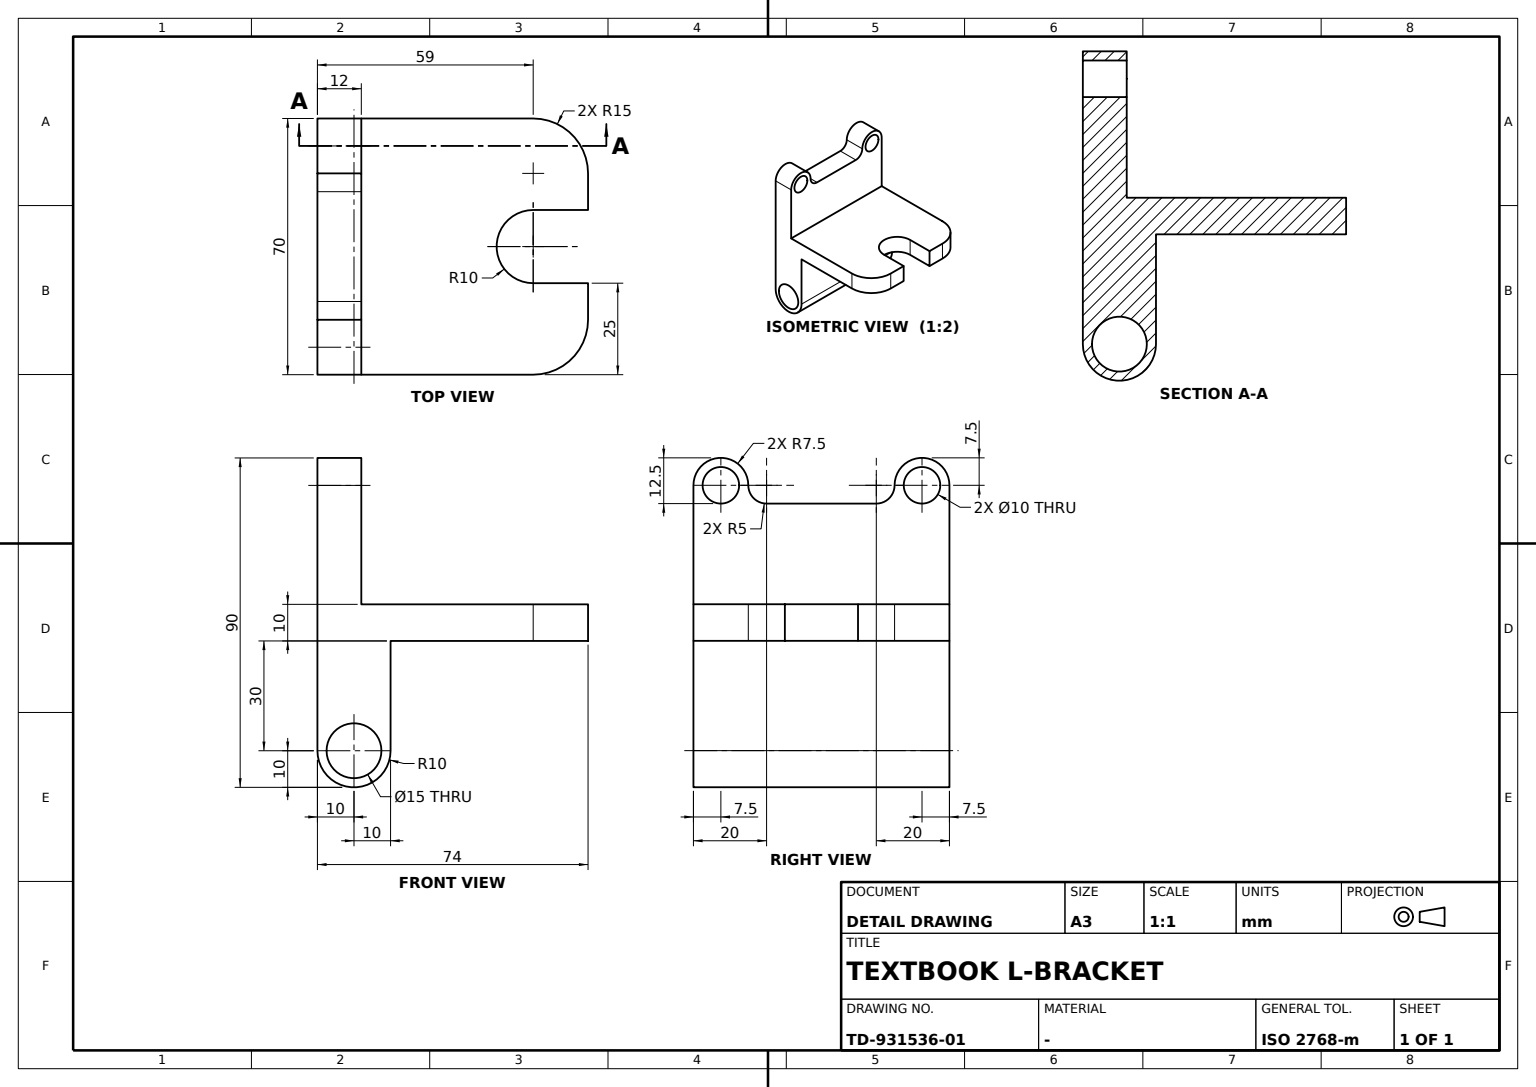
ISO-10303-21;
HEADER;
FILE_DESCRIPTION((''),'2;1');
FILE_NAME('','',(''),(''),'','','');
FILE_SCHEMA(('AUTOMOTIVE_DESIGN'));
ENDSEC;
DATA;
#1=APPLICATION_CONTEXT('');
#2=PRODUCT_CONTEXT('',#1,'mechanical');
#3=PRODUCT('','','',(#2));
#4=PRODUCT_DEFINITION_FORMATION('','',#3);
#5=PRODUCT_DEFINITION_CONTEXT('',#1,'design');
#6=PRODUCT_DEFINITION('','',#4,#5);
#7=PRODUCT_DEFINITION_SHAPE('','',#6);
#8=(LENGTH_UNIT()NAMED_UNIT(*)SI_UNIT(.MILLI.,.METRE.));
#9=(NAMED_UNIT(*)PLANE_ANGLE_UNIT()SI_UNIT($,.RADIAN.));
#10=(NAMED_UNIT(*)SI_UNIT($,.STERADIAN.)SOLID_ANGLE_UNIT());
#11=UNCERTAINTY_MEASURE_WITH_UNIT(LENGTH_MEASURE(1.E-05),#8,'distance_accuracy_value','');
#12=(GEOMETRIC_REPRESENTATION_CONTEXT(3)GLOBAL_UNCERTAINTY_ASSIGNED_CONTEXT((#11))GLOBAL_UNIT_ASSIGNED_CONTEXT((#8,#9,#10))REPRESENTATION_CONTEXT('',''));
#13=CARTESIAN_POINT('',(20.,-6.,37.5));
#14=VERTEX_POINT('',#13);
#15=CARTESIAN_POINT('',(20.,6.,37.5));
#16=VERTEX_POINT('',#15);
#17=CARTESIAN_POINT('',(20.,0.,37.5));
#18=DIRECTION('',(0.,1.,0.));
#19=VECTOR('',#18,1000.);
#20=LINE('',#17,#19);
#21=EDGE_CURVE('',#14,#16,#20,.T.);
#22=ORIENTED_EDGE('',*,*,#21,.F.);
#23=CARTESIAN_POINT('',(35.,-6.,37.5));
#24=VERTEX_POINT('',#23);
#25=CARTESIAN_POINT('',(27.5,-6.,37.5));
#26=DIRECTION('',(-1.,0.,0.));
#27=AXIS2_PLACEMENT_3D('',#25,#18,#26);
#28=CIRCLE('',#27,7.5);
#29=EDGE_CURVE('',#14,#24,#28,.T.);
#30=ORIENTED_EDGE('',*,*,#29,.T.);
#31=CARTESIAN_POINT('',(35.,6.,37.5));
#32=VERTEX_POINT('',#31);
#33=CARTESIAN_POINT('',(35.,0.,37.5));
#34=DIRECTION('',(0.,-1.,0.));
#35=VECTOR('',#34,1000.);
#36=LINE('',#33,#35);
#37=EDGE_CURVE('',#32,#24,#36,.T.);
#38=ORIENTED_EDGE('',*,*,#37,.F.);
#39=CARTESIAN_POINT('',(27.5,6.,37.5));
#40=AXIS2_PLACEMENT_3D('',#39,#18,#26);
#41=CIRCLE('',#40,7.5);
#42=EDGE_CURVE('',#16,#32,#41,.T.);
#43=ORIENTED_EDGE('',*,*,#42,.F.);
#44=EDGE_LOOP('',(#22,#30,#38,#43));
#45=FACE_OUTER_BOUND('',#44,.T.);
#46=CARTESIAN_POINT('',(27.5,0.,37.5));
#47=AXIS2_PLACEMENT_3D('',#46,#34,#26);
#48=CYLINDRICAL_SURFACE('',#47,7.5);
#49=ADVANCED_FACE('',(#45),#48,.T.);
#50=CARTESIAN_POINT('',(-32.5,-6.,37.5));
#51=VERTEX_POINT('',#50);
#52=CARTESIAN_POINT('',(-22.5,-6.,37.5));
#53=VERTEX_POINT('',#52);
#54=CARTESIAN_POINT('',(-27.5,-6.,37.5));
#55=AXIS2_PLACEMENT_3D('',#54,#18,#26);
#56=CIRCLE('',#55,5.);
#57=EDGE_CURVE('',#51,#53,#56,.T.);
#58=ORIENTED_EDGE('',*,*,#57,.F.);
#59=CARTESIAN_POINT('',(-32.5,6.,37.5));
#60=VERTEX_POINT('',#59);
#61=CARTESIAN_POINT('',(-32.5,0.,37.5));
#62=LINE('',#61,#35);
#63=EDGE_CURVE('',#60,#51,#62,.T.);
#64=ORIENTED_EDGE('',*,*,#63,.F.);
#65=CARTESIAN_POINT('',(-22.5,6.,37.5));
#66=VERTEX_POINT('',#65);
#67=CARTESIAN_POINT('',(-27.5,6.,37.5));
#68=AXIS2_PLACEMENT_3D('',#67,#18,#26);
#69=CIRCLE('',#68,5.);
#70=EDGE_CURVE('',#60,#66,#69,.T.);
#71=ORIENTED_EDGE('',*,*,#70,.T.);
#72=CARTESIAN_POINT('',(-22.5,0.,37.5));
#73=LINE('',#72,#35);
#74=EDGE_CURVE('',#66,#53,#73,.T.);
#75=ORIENTED_EDGE('',*,*,#74,.T.);
#76=EDGE_LOOP('',(#58,#64,#71,#75));
#77=FACE_OUTER_BOUND('',#76,.T.);
#78=CARTESIAN_POINT('',(-27.5,0.,37.5));
#79=AXIS2_PLACEMENT_3D('',#78,#34,#26);
#80=CYLINDRICAL_SURFACE('',#79,5.);
#81=ADVANCED_FACE('',(#77),#80,.F.);
#82=CARTESIAN_POINT('',(15.,-6.,32.5));
#83=VERTEX_POINT('',#82);
#84=CARTESIAN_POINT('',(15.,6.,32.5));
#85=VERTEX_POINT('',#84);
#86=CARTESIAN_POINT('',(15.,0.,32.5));
#87=LINE('',#86,#19);
#88=EDGE_CURVE('',#83,#85,#87,.T.);
#89=ORIENTED_EDGE('',*,*,#88,.T.);
#90=CARTESIAN_POINT('',(-15.,6.,32.5));
#91=VERTEX_POINT('',#90);
#92=CARTESIAN_POINT('',(0.,6.,32.5));
#93=VECTOR('',#26,1000.);
#94=LINE('',#92,#93);
#95=EDGE_CURVE('',#85,#91,#94,.T.);
#96=ORIENTED_EDGE('',*,*,#95,.T.);
#97=CARTESIAN_POINT('',(-15.,-6.,32.5));
#98=VERTEX_POINT('',#97);
#99=CARTESIAN_POINT('',(-15.,0.,32.5));
#100=LINE('',#99,#19);
#101=EDGE_CURVE('',#98,#91,#100,.T.);
#102=ORIENTED_EDGE('',*,*,#101,.F.);
#103=CARTESIAN_POINT('',(0.,-6.,32.5));
#104=DIRECTION('',(1.,0.,0.));
#105=VECTOR('',#104,1000.);
#106=LINE('',#103,#105);
#107=EDGE_CURVE('',#98,#83,#106,.T.);
#108=ORIENTED_EDGE('',*,*,#107,.T.);
#109=EDGE_LOOP('',(#89,#96,#102,#108));
#110=FACE_OUTER_BOUND('',#109,.T.);
#111=CARTESIAN_POINT('',(-27.5,6.,32.5));
#112=DIRECTION('',(0.,0.,-1.));
#113=AXIS2_PLACEMENT_3D('',#111,#112,#104);
#114=PLANE('',#113);
#115=ADVANCED_FACE('',(#110),#114,.F.);
#116=CARTESIAN_POINT('',(-10.,53.,-5.));
#117=VERTEX_POINT('',#116);
#118=CARTESIAN_POINT('',(10.,53.,-5.));
#119=VERTEX_POINT('',#118);
#120=CARTESIAN_POINT('',(0.,53.,-5.));
#121=DIRECTION('',(0.,0.,1.));
#122=AXIS2_PLACEMENT_3D('',#120,#121,#34);
#123=CIRCLE('',#122,10.);
#124=EDGE_CURVE('',#117,#119,#123,.T.);
#125=ORIENTED_EDGE('',*,*,#124,.T.);
#126=CARTESIAN_POINT('',(10.,68.,-5.));
#127=VERTEX_POINT('',#126);
#128=CARTESIAN_POINT('',(10.,60.5,-5.));
#129=LINE('',#128,#35);
#130=EDGE_CURVE('',#127,#119,#129,.T.);
#131=ORIENTED_EDGE('',*,*,#130,.F.);
#132=CARTESIAN_POINT('',(20.,68.,-5.));
#133=VERTEX_POINT('',#132);
#134=CARTESIAN_POINT('',(15.,68.,-5.));
#135=LINE('',#134,#105);
#136=EDGE_CURVE('',#127,#133,#135,.T.);
#137=ORIENTED_EDGE('',*,*,#136,.T.);
#138=CARTESIAN_POINT('',(35.,53.,-5.));
#139=VERTEX_POINT('',#138);
#140=CARTESIAN_POINT('',(20.,53.,-5.));
#141=AXIS2_PLACEMENT_3D('',#140,#121,#34);
#142=CIRCLE('',#141,15.);
#143=EDGE_CURVE('',#139,#133,#142,.T.);
#144=ORIENTED_EDGE('',*,*,#143,.F.);
#145=CARTESIAN_POINT('',(35.,14.,-5.));
#146=VERTEX_POINT('',#145);
#147=CARTESIAN_POINT('',(35.,33.5,-5.));
#148=LINE('',#147,#19);
#149=EDGE_CURVE('',#146,#139,#148,.T.);
#150=ORIENTED_EDGE('',*,*,#149,.F.);
#151=CARTESIAN_POINT('',(-35.,14.,-5.));
#152=VERTEX_POINT('',#151);
#153=CARTESIAN_POINT('',(0.,14.,-5.));
#154=LINE('',#153,#105);
#155=EDGE_CURVE('',#152,#146,#154,.T.);
#156=ORIENTED_EDGE('',*,*,#155,.F.);
#157=CARTESIAN_POINT('',(-35.,53.,-5.));
#158=VERTEX_POINT('',#157);
#159=CARTESIAN_POINT('',(-35.,33.5,-5.));
#160=LINE('',#159,#19);
#161=EDGE_CURVE('',#152,#158,#160,.T.);
#162=ORIENTED_EDGE('',*,*,#161,.T.);
#163=CARTESIAN_POINT('',(-20.,68.,-5.));
#164=VERTEX_POINT('',#163);
#165=CARTESIAN_POINT('',(-20.,53.,-5.));
#166=AXIS2_PLACEMENT_3D('',#165,#121,#34);
#167=CIRCLE('',#166,15.);
#168=EDGE_CURVE('',#164,#158,#167,.T.);
#169=ORIENTED_EDGE('',*,*,#168,.F.);
#170=CARTESIAN_POINT('',(-10.,68.,-5.));
#171=VERTEX_POINT('',#170);
#172=CARTESIAN_POINT('',(-15.,68.,-5.));
#173=LINE('',#172,#105);
#174=EDGE_CURVE('',#164,#171,#173,.T.);
#175=ORIENTED_EDGE('',*,*,#174,.T.);
#176=CARTESIAN_POINT('',(-10.,60.5,-5.));
#177=LINE('',#176,#35);
#178=EDGE_CURVE('',#171,#117,#177,.T.);
#179=ORIENTED_EDGE('',*,*,#178,.T.);
#180=EDGE_LOOP('',(#125,#131,#137,#144,#150,#156,#162,#169,#175,#179));
#181=FACE_OUTER_BOUND('',#180,.T.);
#182=CARTESIAN_POINT('',(0.,68.,-5.));
#183=AXIS2_PLACEMENT_3D('',#182,#121,#34);
#184=PLANE('',#183);
#185=ADVANCED_FACE('',(#181),#184,.F.);
#186=CARTESIAN_POINT('',(10.,68.,5.));
#187=VERTEX_POINT('',#186);
#188=CARTESIAN_POINT('',(10.,68.,0.));
#189=VECTOR('',#112,1000.);
#190=LINE('',#188,#189);
#191=EDGE_CURVE('',#187,#127,#190,.T.);
#192=ORIENTED_EDGE('',*,*,#191,.F.);
#193=CARTESIAN_POINT('',(20.,68.,5.));
#194=VERTEX_POINT('',#193);
#195=CARTESIAN_POINT('',(15.,68.,5.));
#196=LINE('',#195,#105);
#197=EDGE_CURVE('',#187,#194,#196,.T.);
#198=ORIENTED_EDGE('',*,*,#197,.T.);
#199=CARTESIAN_POINT('',(20.,68.,0.));
#200=VECTOR('',#121,1000.);
#201=LINE('',#199,#200);
#202=EDGE_CURVE('',#133,#194,#201,.T.);
#203=ORIENTED_EDGE('',*,*,#202,.F.);
#204=ORIENTED_EDGE('',*,*,#136,.F.);
#205=EDGE_LOOP('',(#192,#198,#203,#204));
#206=FACE_OUTER_BOUND('',#205,.T.);
#207=CARTESIAN_POINT('',(0.,68.,5.));
#208=AXIS2_PLACEMENT_3D('',#207,#34,#112);
#209=PLANE('',#208);
#210=ADVANCED_FACE('',(#206),#209,.F.);
#211=ORIENTED_EDGE('',*,*,#143,.T.);
#212=ORIENTED_EDGE('',*,*,#202,.T.);
#213=CARTESIAN_POINT('',(35.,53.,5.));
#214=VERTEX_POINT('',#213);
#215=CARTESIAN_POINT('',(20.,53.,5.));
#216=AXIS2_PLACEMENT_3D('',#215,#112,#18);
#217=CIRCLE('',#216,15.);
#218=EDGE_CURVE('',#194,#214,#217,.T.);
#219=ORIENTED_EDGE('',*,*,#218,.T.);
#220=CARTESIAN_POINT('',(35.,53.,0.));
#221=LINE('',#220,#200);
#222=EDGE_CURVE('',#139,#214,#221,.T.);
#223=ORIENTED_EDGE('',*,*,#222,.F.);
#224=EDGE_LOOP('',(#211,#212,#219,#223));
#225=FACE_OUTER_BOUND('',#224,.T.);
#226=CARTESIAN_POINT('',(20.,53.,-3.75));
#227=AXIS2_PLACEMENT_3D('',#226,#121,#18);
#228=CYLINDRICAL_SURFACE('',#227,15.);
#229=ADVANCED_FACE('',(#225),#228,.T.);
#230=CARTESIAN_POINT('',(-10.,53.,5.));
#231=VERTEX_POINT('',#230);
#232=CARTESIAN_POINT('',(-10.,53.,0.));
#233=LINE('',#232,#189);
#234=EDGE_CURVE('',#231,#117,#233,.T.);
#235=ORIENTED_EDGE('',*,*,#234,.T.);
#236=ORIENTED_EDGE('',*,*,#178,.F.);
#237=CARTESIAN_POINT('',(-10.,68.,5.));
#238=VERTEX_POINT('',#237);
#239=CARTESIAN_POINT('',(-10.,68.,0.));
#240=LINE('',#239,#189);
#241=EDGE_CURVE('',#238,#171,#240,.T.);
#242=ORIENTED_EDGE('',*,*,#241,.F.);
#243=CARTESIAN_POINT('',(-10.,60.5,5.));
#244=LINE('',#243,#35);
#245=EDGE_CURVE('',#238,#231,#244,.T.);
#246=ORIENTED_EDGE('',*,*,#245,.T.);
#247=EDGE_LOOP('',(#235,#236,#242,#246));
#248=FACE_OUTER_BOUND('',#247,.T.);
#249=AXIS2_PLACEMENT_3D('',#230,#26,#18);
#250=PLANE('',#249);
#251=ADVANCED_FACE('',(#248),#250,.F.);
#252=ORIENTED_EDGE('',*,*,#174,.F.);
#253=CARTESIAN_POINT('',(-20.,68.,5.));
#254=VERTEX_POINT('',#253);
#255=CARTESIAN_POINT('',(-20.,68.,0.));
#256=LINE('',#255,#200);
#257=EDGE_CURVE('',#164,#254,#256,.T.);
#258=ORIENTED_EDGE('',*,*,#257,.T.);
#259=CARTESIAN_POINT('',(-15.,68.,5.));
#260=LINE('',#259,#105);
#261=EDGE_CURVE('',#254,#238,#260,.T.);
#262=ORIENTED_EDGE('',*,*,#261,.T.);
#263=ORIENTED_EDGE('',*,*,#241,.T.);
#264=EDGE_LOOP('',(#252,#258,#262,#263));
#265=FACE_OUTER_BOUND('',#264,.T.);
#266=ADVANCED_FACE('',(#265),#209,.F.);
#267=CARTESIAN_POINT('',(-35.,-6.,-35.));
#268=VERTEX_POINT('',#267);
#269=CARTESIAN_POINT('',(-35.,14.,-35.));
#270=VERTEX_POINT('',#269);
#271=CARTESIAN_POINT('',(-35.,4.,-35.));
#272=AXIS2_PLACEMENT_3D('',#271,#104,#18);
#273=CIRCLE('',#272,10.);
#274=EDGE_CURVE('',#268,#270,#273,.T.);
#275=ORIENTED_EDGE('',*,*,#274,.T.);
#276=CARTESIAN_POINT('',(35.,14.,-35.));
#277=VERTEX_POINT('',#276);
#278=CARTESIAN_POINT('',(0.,14.,-35.));
#279=LINE('',#278,#105);
#280=EDGE_CURVE('',#270,#277,#279,.T.);
#281=ORIENTED_EDGE('',*,*,#280,.T.);
#282=CARTESIAN_POINT('',(35.,-6.,-35.));
#283=VERTEX_POINT('',#282);
#284=CARTESIAN_POINT('',(35.,4.,-35.));
#285=AXIS2_PLACEMENT_3D('',#284,#104,#18);
#286=CIRCLE('',#285,10.);
#287=EDGE_CURVE('',#283,#277,#286,.T.);
#288=ORIENTED_EDGE('',*,*,#287,.F.);
#289=CARTESIAN_POINT('',(0.,-6.,-35.));
#290=LINE('',#289,#105);
#291=EDGE_CURVE('',#268,#283,#290,.T.);
#292=ORIENTED_EDGE('',*,*,#291,.F.);
#293=EDGE_LOOP('',(#275,#281,#288,#292));
#294=FACE_OUTER_BOUND('',#293,.T.);
#295=CARTESIAN_POINT('',(0.,4.,-35.));
#296=AXIS2_PLACEMENT_3D('',#295,#26,#18);
#297=CYLINDRICAL_SURFACE('',#296,10.);
#298=ADVANCED_FACE('',(#294),#297,.T.);
#299=CARTESIAN_POINT('',(15.,6.,37.5));
#300=AXIS2_PLACEMENT_3D('',#299,#34,#121);
#301=CIRCLE('',#300,5.);
#302=EDGE_CURVE('',#85,#16,#301,.T.);
#303=ORIENTED_EDGE('',*,*,#302,.F.);
#304=ORIENTED_EDGE('',*,*,#88,.F.);
#305=CARTESIAN_POINT('',(15.,-6.,37.5));
#306=AXIS2_PLACEMENT_3D('',#305,#18,#112);
#307=CIRCLE('',#306,5.);
#308=EDGE_CURVE('',#14,#83,#307,.T.);
#309=ORIENTED_EDGE('',*,*,#308,.F.);
#310=ORIENTED_EDGE('',*,*,#21,.T.);
#311=EDGE_LOOP('',(#303,#304,#309,#310));
#312=FACE_OUTER_BOUND('',#311,.T.);
#313=CARTESIAN_POINT('',(15.,0.,37.5));
#314=AXIS2_PLACEMENT_3D('',#313,#34,#112);
#315=CYLINDRICAL_SURFACE('',#314,5.);
#316=ADVANCED_FACE('',(#312),#315,.F.);
#317=CARTESIAN_POINT('',(-20.,-6.,37.5));
#318=VERTEX_POINT('',#317);
#319=CARTESIAN_POINT('',(-20.,6.,37.5));
#320=VERTEX_POINT('',#319);
#321=CARTESIAN_POINT('',(-20.,0.,37.5));
#322=LINE('',#321,#19);
#323=EDGE_CURVE('',#318,#320,#322,.T.);
#324=ORIENTED_EDGE('',*,*,#323,.T.);
#325=CARTESIAN_POINT('',(-35.,6.,37.5));
#326=VERTEX_POINT('',#325);
#327=CIRCLE('',#68,7.5);
#328=EDGE_CURVE('',#326,#320,#327,.T.);
#329=ORIENTED_EDGE('',*,*,#328,.F.);
#330=CARTESIAN_POINT('',(-35.,-6.,37.5));
#331=VERTEX_POINT('',#330);
#332=CARTESIAN_POINT('',(-35.,0.,37.5));
#333=LINE('',#332,#35);
#334=EDGE_CURVE('',#326,#331,#333,.T.);
#335=ORIENTED_EDGE('',*,*,#334,.T.);
#336=CIRCLE('',#55,7.5);
#337=EDGE_CURVE('',#331,#318,#336,.T.);
#338=ORIENTED_EDGE('',*,*,#337,.T.);
#339=EDGE_LOOP('',(#324,#329,#335,#338));
#340=FACE_OUTER_BOUND('',#339,.T.);
#341=CYLINDRICAL_SURFACE('',#79,7.5);
#342=ADVANCED_FACE('',(#340),#341,.T.);
#343=CARTESIAN_POINT('',(32.5,6.,37.5));
#344=VERTEX_POINT('',#343);
#345=CARTESIAN_POINT('',(32.5,-6.,37.5));
#346=VERTEX_POINT('',#345);
#347=CARTESIAN_POINT('',(32.5,0.,37.5));
#348=LINE('',#347,#35);
#349=EDGE_CURVE('',#344,#346,#348,.T.);
#350=ORIENTED_EDGE('',*,*,#349,.F.);
#351=CARTESIAN_POINT('',(22.5,6.,37.5));
#352=VERTEX_POINT('',#351);
#353=CIRCLE('',#40,5.);
#354=EDGE_CURVE('',#344,#352,#353,.T.);
#355=ORIENTED_EDGE('',*,*,#354,.T.);
#356=CARTESIAN_POINT('',(22.5,-6.,37.5));
#357=VERTEX_POINT('',#356);
#358=CARTESIAN_POINT('',(22.5,0.,37.5));
#359=LINE('',#358,#35);
#360=EDGE_CURVE('',#352,#357,#359,.T.);
#361=ORIENTED_EDGE('',*,*,#360,.T.);
#362=CIRCLE('',#27,5.);
#363=EDGE_CURVE('',#346,#357,#362,.T.);
#364=ORIENTED_EDGE('',*,*,#363,.F.);
#365=EDGE_LOOP('',(#350,#355,#361,#364));
#366=FACE_OUTER_BOUND('',#365,.T.);
#367=CYLINDRICAL_SURFACE('',#47,5.);
#368=ADVANCED_FACE('',(#366),#367,.F.);
#369=ORIENTED_EDGE('',*,*,#280,.F.);
#370=CARTESIAN_POINT('',(-35.,14.,-20.));
#371=LINE('',#370,#200);
#372=EDGE_CURVE('',#270,#152,#371,.T.);
#373=ORIENTED_EDGE('',*,*,#372,.T.);
#374=ORIENTED_EDGE('',*,*,#155,.T.);
#375=CARTESIAN_POINT('',(35.,14.,-20.));
#376=LINE('',#375,#200);
#377=EDGE_CURVE('',#277,#146,#376,.T.);
#378=ORIENTED_EDGE('',*,*,#377,.F.);
#379=EDGE_LOOP('',(#369,#373,#374,#378));
#380=FACE_OUTER_BOUND('',#379,.T.);
#381=AXIS2_PLACEMENT_3D('',#278,#18,#121);
#382=PLANE('',#381);
#383=ADVANCED_FACE('',(#380),#382,.T.);
#384=CARTESIAN_POINT('',(-35.,11.5,-35.));
#385=VERTEX_POINT('',#384);
#386=CARTESIAN_POINT('',(-35.,-3.5,-35.));
#387=VERTEX_POINT('',#386);
#388=CIRCLE('',#272,7.5);
#389=EDGE_CURVE('',#385,#387,#388,.T.);
#390=ORIENTED_EDGE('',*,*,#389,.T.);
#391=EDGE_CURVE('',#387,#385,#388,.T.);
#392=ORIENTED_EDGE('',*,*,#391,.T.);
#393=EDGE_LOOP('',(#390,#392));
#394=FACE_BOUND('',#393,.T.);
#395=CARTESIAN_POINT('',(-35.,53.,5.));
#396=VERTEX_POINT('',#395);
#397=CARTESIAN_POINT('',(-35.,53.,0.));
#398=LINE('',#397,#200);
#399=EDGE_CURVE('',#158,#396,#398,.T.);
#400=ORIENTED_EDGE('',*,*,#399,.F.);
#401=ORIENTED_EDGE('',*,*,#161,.F.);
#402=ORIENTED_EDGE('',*,*,#372,.F.);
#403=ORIENTED_EDGE('',*,*,#274,.F.);
#404=CARTESIAN_POINT('',(-35.,-6.,1.25));
#405=LINE('',#404,#189);
#406=EDGE_CURVE('',#331,#268,#405,.T.);
#407=ORIENTED_EDGE('',*,*,#406,.F.);
#408=ORIENTED_EDGE('',*,*,#334,.F.);
#409=CARTESIAN_POINT('',(-35.,6.,5.));
#410=VERTEX_POINT('',#409);
#411=CARTESIAN_POINT('',(-35.,6.,21.25));
#412=LINE('',#411,#200);
#413=EDGE_CURVE('',#410,#326,#412,.T.);
#414=ORIENTED_EDGE('',*,*,#413,.F.);
#415=CARTESIAN_POINT('',(-35.,29.5,5.));
#416=LINE('',#415,#35);
#417=EDGE_CURVE('',#396,#410,#416,.T.);
#418=ORIENTED_EDGE('',*,*,#417,.F.);
#419=EDGE_LOOP('',(#400,#401,#402,#403,#407,#408,#414,#418));
#420=FACE_OUTER_BOUND('',#419,.T.);
#421=CARTESIAN_POINT('',(-35.,0.,0.));
#422=AXIS2_PLACEMENT_3D('',#421,#104,#18);
#423=PLANE('',#422);
#424=ADVANCED_FACE('',(#394,#420),#423,.F.);
#425=CARTESIAN_POINT('',(35.,11.5,-35.));
#426=VERTEX_POINT('',#425);
#427=CARTESIAN_POINT('',(0.,11.5,-35.));
#428=LINE('',#427,#93);
#429=EDGE_CURVE('',#426,#385,#428,.T.);
#430=ORIENTED_EDGE('',*,*,#429,.T.);
#431=ORIENTED_EDGE('',*,*,#391,.F.);
#432=CARTESIAN_POINT('',(35.,-3.5,-35.));
#433=VERTEX_POINT('',#432);
#434=CARTESIAN_POINT('',(0.,-3.5,-35.));
#435=LINE('',#434,#93);
#436=EDGE_CURVE('',#433,#387,#435,.T.);
#437=ORIENTED_EDGE('',*,*,#436,.F.);
#438=CIRCLE('',#285,7.5);
#439=EDGE_CURVE('',#433,#426,#438,.T.);
#440=ORIENTED_EDGE('',*,*,#439,.T.);
#441=EDGE_LOOP('',(#430,#431,#437,#440));
#442=FACE_OUTER_BOUND('',#441,.T.);
#443=CYLINDRICAL_SURFACE('',#296,7.5);
#444=ADVANCED_FACE('',(#442),#443,.F.);
#445=CARTESIAN_POINT('',(35.,6.,5.));
#446=VERTEX_POINT('',#445);
#447=CARTESIAN_POINT('',(35.,6.,21.25));
#448=LINE('',#447,#200);
#449=EDGE_CURVE('',#446,#32,#448,.T.);
#450=ORIENTED_EDGE('',*,*,#449,.T.);
#451=ORIENTED_EDGE('',*,*,#37,.T.);
#452=CARTESIAN_POINT('',(35.,-6.,1.25));
#453=LINE('',#452,#189);
#454=EDGE_CURVE('',#24,#283,#453,.T.);
#455=ORIENTED_EDGE('',*,*,#454,.T.);
#456=ORIENTED_EDGE('',*,*,#287,.T.);
#457=ORIENTED_EDGE('',*,*,#377,.T.);
#458=ORIENTED_EDGE('',*,*,#149,.T.);
#459=ORIENTED_EDGE('',*,*,#222,.T.);
#460=CARTESIAN_POINT('',(35.,29.5,5.));
#461=LINE('',#460,#35);
#462=EDGE_CURVE('',#214,#446,#461,.T.);
#463=ORIENTED_EDGE('',*,*,#462,.T.);
#464=EDGE_LOOP('',(#450,#451,#455,#456,#457,#458,#459,#463));
#465=FACE_OUTER_BOUND('',#464,.T.);
#466=EDGE_CURVE('',#426,#433,#438,.T.);
#467=ORIENTED_EDGE('',*,*,#466,.F.);
#468=ORIENTED_EDGE('',*,*,#439,.F.);
#469=EDGE_LOOP('',(#467,#468));
#470=FACE_BOUND('',#469,.T.);
#471=CARTESIAN_POINT('',(35.,0.,0.));
#472=AXIS2_PLACEMENT_3D('',#471,#104,#18);
#473=PLANE('',#472);
#474=ADVANCED_FACE('',(#465,#470),#473,.T.);
#475=ORIENTED_EDGE('',*,*,#101,.T.);
#476=CARTESIAN_POINT('',(-15.,6.,37.5));
#477=AXIS2_PLACEMENT_3D('',#476,#34,#121);
#478=CIRCLE('',#477,5.);
#479=EDGE_CURVE('',#320,#91,#478,.T.);
#480=ORIENTED_EDGE('',*,*,#479,.F.);
#481=ORIENTED_EDGE('',*,*,#323,.F.);
#482=CARTESIAN_POINT('',(-15.,-6.,37.5));
#483=AXIS2_PLACEMENT_3D('',#482,#18,#112);
#484=CIRCLE('',#483,5.);
#485=EDGE_CURVE('',#98,#318,#484,.T.);
#486=ORIENTED_EDGE('',*,*,#485,.F.);
#487=EDGE_LOOP('',(#475,#480,#481,#486));
#488=FACE_OUTER_BOUND('',#487,.T.);
#489=CARTESIAN_POINT('',(-15.,0.,37.5));
#490=AXIS2_PLACEMENT_3D('',#489,#34,#26);
#491=CYLINDRICAL_SURFACE('',#490,5.);
#492=ADVANCED_FACE('',(#488),#491,.F.);
#493=ORIENTED_EDGE('',*,*,#354,.F.);
#494=EDGE_CURVE('',#352,#344,#353,.T.);
#495=ORIENTED_EDGE('',*,*,#494,.F.);
#496=EDGE_LOOP('',(#493,#495));
#497=FACE_BOUND('',#496,.T.);
#498=ORIENTED_EDGE('',*,*,#70,.F.);
#499=EDGE_CURVE('',#66,#60,#69,.T.);
#500=ORIENTED_EDGE('',*,*,#499,.F.);
#501=EDGE_LOOP('',(#498,#500));
#502=FACE_BOUND('',#501,.T.);
#503=ORIENTED_EDGE('',*,*,#328,.T.);
#504=ORIENTED_EDGE('',*,*,#479,.T.);
#505=ORIENTED_EDGE('',*,*,#95,.F.);
#506=ORIENTED_EDGE('',*,*,#302,.T.);
#507=ORIENTED_EDGE('',*,*,#42,.T.);
#508=ORIENTED_EDGE('',*,*,#449,.F.);
#509=CARTESIAN_POINT('',(0.,6.,5.));
#510=LINE('',#509,#105);
#511=EDGE_CURVE('',#410,#446,#510,.T.);
#512=ORIENTED_EDGE('',*,*,#511,.F.);
#513=ORIENTED_EDGE('',*,*,#413,.T.);
#514=EDGE_LOOP('',(#503,#504,#505,#506,#507,#508,#512,#513));
#515=FACE_OUTER_BOUND('',#514,.T.);
#516=AXIS2_PLACEMENT_3D('',#509,#18,#121);
#517=PLANE('',#516);
#518=ADVANCED_FACE('',(#497,#502,#515),#517,.T.);
#519=ORIENTED_EDGE('',*,*,#257,.F.);
#520=ORIENTED_EDGE('',*,*,#168,.T.);
#521=ORIENTED_EDGE('',*,*,#399,.T.);
#522=CARTESIAN_POINT('',(-20.,53.,5.));
#523=AXIS2_PLACEMENT_3D('',#522,#112,#18);
#524=CIRCLE('',#523,15.);
#525=EDGE_CURVE('',#396,#254,#524,.T.);
#526=ORIENTED_EDGE('',*,*,#525,.T.);
#527=EDGE_LOOP('',(#519,#520,#521,#526));
#528=FACE_OUTER_BOUND('',#527,.T.);
#529=CARTESIAN_POINT('',(-20.,53.,-3.75));
#530=AXIS2_PLACEMENT_3D('',#529,#121,#26);
#531=CYLINDRICAL_SURFACE('',#530,15.);
#532=ADVANCED_FACE('',(#528),#531,.T.);
#533=ORIENTED_EDGE('',*,*,#74,.F.);
#534=ORIENTED_EDGE('',*,*,#499,.T.);
#535=ORIENTED_EDGE('',*,*,#63,.T.);
#536=EDGE_CURVE('',#53,#51,#56,.T.);
#537=ORIENTED_EDGE('',*,*,#536,.F.);
#538=EDGE_LOOP('',(#533,#534,#535,#537));
#539=FACE_OUTER_BOUND('',#538,.T.);
#540=ADVANCED_FACE('',(#539),#80,.F.);
#541=CARTESIAN_POINT('',(10.,53.,5.));
#542=VERTEX_POINT('',#541);
#543=CARTESIAN_POINT('',(10.,60.5,5.));
#544=LINE('',#543,#19);
#545=EDGE_CURVE('',#542,#187,#544,.T.);
#546=ORIENTED_EDGE('',*,*,#545,.T.);
#547=ORIENTED_EDGE('',*,*,#191,.T.);
#548=ORIENTED_EDGE('',*,*,#130,.T.);
#549=CARTESIAN_POINT('',(10.,53.,-30.));
#550=LINE('',#549,#189);
#551=EDGE_CURVE('',#542,#119,#550,.T.);
#552=ORIENTED_EDGE('',*,*,#551,.F.);
#553=EDGE_LOOP('',(#546,#547,#548,#552));
#554=FACE_OUTER_BOUND('',#553,.T.);
#555=AXIS2_PLACEMENT_3D('',#186,#104,#34);
#556=PLANE('',#555);
#557=ADVANCED_FACE('',(#554),#556,.F.);
#558=ORIENTED_EDGE('',*,*,#429,.F.);
#559=ORIENTED_EDGE('',*,*,#466,.T.);
#560=ORIENTED_EDGE('',*,*,#436,.T.);
#561=ORIENTED_EDGE('',*,*,#389,.F.);
#562=EDGE_LOOP('',(#558,#559,#560,#561));
#563=FACE_OUTER_BOUND('',#562,.T.);
#564=ADVANCED_FACE('',(#563),#443,.F.);
#565=ORIENTED_EDGE('',*,*,#545,.F.);
#566=CARTESIAN_POINT('',(0.,53.,5.));
#567=AXIS2_PLACEMENT_3D('',#566,#121,#104);
#568=CIRCLE('',#567,10.);
#569=EDGE_CURVE('',#231,#542,#568,.T.);
#570=ORIENTED_EDGE('',*,*,#569,.F.);
#571=ORIENTED_EDGE('',*,*,#245,.F.);
#572=ORIENTED_EDGE('',*,*,#261,.F.);
#573=ORIENTED_EDGE('',*,*,#525,.F.);
#574=ORIENTED_EDGE('',*,*,#417,.T.);
#575=ORIENTED_EDGE('',*,*,#511,.T.);
#576=ORIENTED_EDGE('',*,*,#462,.F.);
#577=ORIENTED_EDGE('',*,*,#218,.F.);
#578=ORIENTED_EDGE('',*,*,#197,.F.);
#579=EDGE_LOOP('',(#565,#570,#571,#572,#573,#574,#575,#576,#577,#578));
#580=FACE_OUTER_BOUND('',#579,.T.);
#581=AXIS2_PLACEMENT_3D('',#509,#112,#18);
#582=PLANE('',#581);
#583=ADVANCED_FACE('',(#580),#582,.F.);
#584=ORIENTED_EDGE('',*,*,#349,.T.);
#585=EDGE_CURVE('',#357,#346,#362,.T.);
#586=ORIENTED_EDGE('',*,*,#585,.F.);
#587=ORIENTED_EDGE('',*,*,#360,.F.);
#588=ORIENTED_EDGE('',*,*,#494,.T.);
#589=EDGE_LOOP('',(#584,#586,#587,#588));
#590=FACE_OUTER_BOUND('',#589,.T.);
#591=ADVANCED_FACE('',(#590),#367,.F.);
#592=ORIENTED_EDGE('',*,*,#585,.T.);
#593=ORIENTED_EDGE('',*,*,#363,.T.);
#594=EDGE_LOOP('',(#592,#593));
#595=FACE_BOUND('',#594,.T.);
#596=ORIENTED_EDGE('',*,*,#454,.F.);
#597=ORIENTED_EDGE('',*,*,#29,.F.);
#598=ORIENTED_EDGE('',*,*,#308,.T.);
#599=ORIENTED_EDGE('',*,*,#107,.F.);
#600=ORIENTED_EDGE('',*,*,#485,.T.);
#601=ORIENTED_EDGE('',*,*,#337,.F.);
#602=ORIENTED_EDGE('',*,*,#406,.T.);
#603=ORIENTED_EDGE('',*,*,#291,.T.);
#604=EDGE_LOOP('',(#596,#597,#598,#599,#600,#601,#602,#603));
#605=FACE_OUTER_BOUND('',#604,.T.);
#606=ORIENTED_EDGE('',*,*,#57,.T.);
#607=ORIENTED_EDGE('',*,*,#536,.T.);
#608=EDGE_LOOP('',(#606,#607));
#609=FACE_BOUND('',#608,.T.);
#610=CARTESIAN_POINT('',(0.,-6.,37.5));
#611=AXIS2_PLACEMENT_3D('',#610,#34,#112);
#612=PLANE('',#611);
#613=ADVANCED_FACE('',(#595,#605,#609),#612,.T.);
#614=ORIENTED_EDGE('',*,*,#569,.T.);
#615=ORIENTED_EDGE('',*,*,#551,.T.);
#616=ORIENTED_EDGE('',*,*,#124,.F.);
#617=ORIENTED_EDGE('',*,*,#234,.F.);
#618=EDGE_LOOP('',(#614,#615,#616,#617));
#619=FACE_OUTER_BOUND('',#618,.T.);
#620=CARTESIAN_POINT('',(0.,53.,-30.));
#621=AXIS2_PLACEMENT_3D('',#620,#112,#104);
#622=CYLINDRICAL_SURFACE('',#621,10.);
#623=ADVANCED_FACE('',(#619),#622,.F.);
#624=CLOSED_SHELL('',(#49,#81,#115,#185,#210,#229,#251,#266,#298,#316,#342,#368,#383,#424,#444,#474,#492,#518,#532,#540,#557,#564,#583,#591,#613,#623));
#625=MANIFOLD_SOLID_BREP('',#624);
#626=ADVANCED_BREP_SHAPE_REPRESENTATION('',(#625),#12);
#627=SHAPE_DEFINITION_REPRESENTATION(#7,#626);
ENDSEC;
END-ISO-10303-21;
